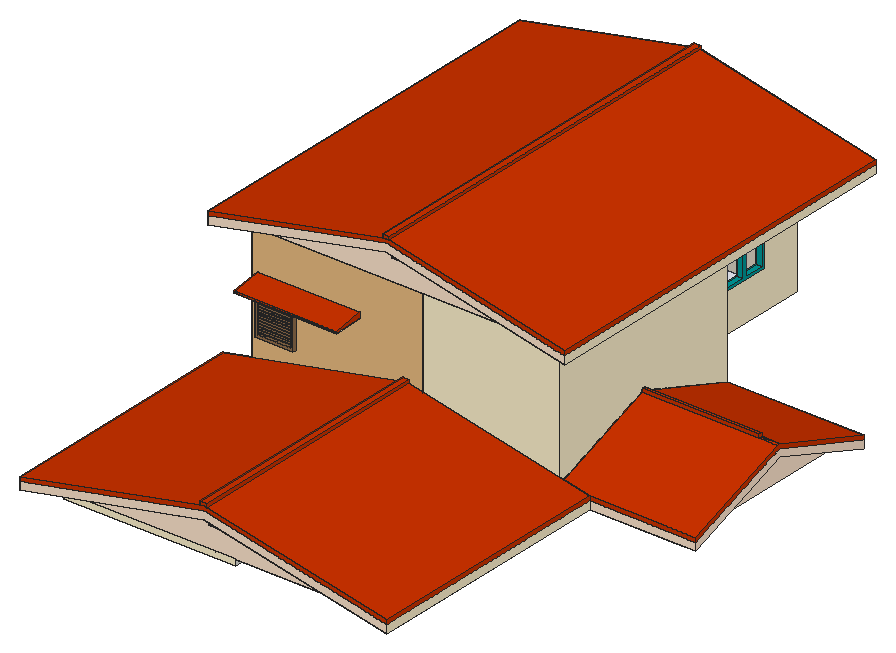
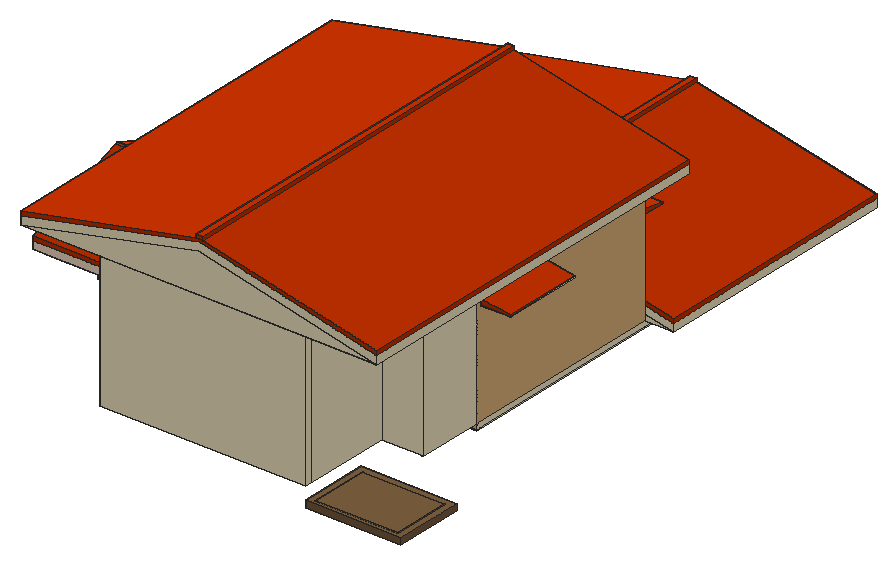
# SketchUp Ruby script. Lengths in inches.
U = 1.inch
M = Sketchup.active_model
def pt(a) = Geom::Point3d.new(a.map { |v| v * U })
def face(e, loops, mat)
  f = e.add_face(loops[0].map { |a| pt(a) })
  loops[1..].each { |l| e.add_face(l.map { |a| pt(a) }).erase! }
  f.material = f.back_material = mat if mat
  f
end
# faces: each face lists its corners as indices into pts; further lists are holes
def faces(e, pts, list, mat = nil) = list.each { |f| face(e, (f[0].is_a?(Array) ? f : [f]).map { |l| l.map { |i| pts[i] } }, mat) }
# xy, xz, yz: faces in a plane at the given z, y or x. An outline is a flat list of corners, or four numbers for a rectangle; further outlines are holes
def ring(l) = l.size == 4 ? [[l[0], l[1]], [l[2], l[1]], [l[2], l[3]], [l[0], l[3]]] : l.each_slice(2).to_a
def flat(e, list, mat, &to3) = list.each { |f| face(e, (f[0].is_a?(Array) ? f : [f]).map { |l| ring(l).map { |u, v| to3.(u, v) } }, mat) }
def xy(e, z, list, mat = nil) = flat(e, list, mat) { |x, y| [x, y, z] }
def xz(e, y, list, mat = nil) = flat(e, list, mat) { |x, z| [x, y, z] }
def yz(e, x, list, mat = nil) = flat(e, list, mat) { |y, z| [x, y, z] }
def lines(e, pts, list) = list.each { |a, b| e.add_line(pt(pts[a]), pt(pts[b])) }
# prism: a flat outline (further loops are holes) pulled along v
def prism(e, loops, v, mat = nil)
  f = face(e, loops, mat); d = Geom::Vector3d.new(v.map { |x| x * U })
  f.pushpull(f.normal.samedirection?(d) ? d.length : -d.length)
end
def box(e, o, s, mat = nil) = prism(e, [[o, [o[0] + s[0], o[1], o[2]], [o[0] + s[0], o[1] + s[1], o[2]], [o[0], o[1] + s[1], o[2]]]], [0, 0, s[2]], mat)
def at(x, y, z, deg = 0) = Geom::Transformation.translation(pt([x, y, z])) * Geom::Transformation.rotation(ORIGIN, Z_AXIS, deg.degrees)
def axes(o, x, y, z) = Geom::Transformation.new([*x, 0, *y, 0, *z, 0, *pt(o).to_a, 1])
def part(name) = M.definitions.add(name)
# library, detail: a bought-in or finely detailed component or shape, given as its bounding box
def library(name, o, s) = part(name).tap { |d| box(d.entities, o, s) }
def detail(e, o, s) = box(e.add_group.entities, o, s)
def put(e, d, t, mat = nil) = e.add_instance(d, t).tap { |i| i.material = mat if mat }
def group(e, t, mat = nil) = e.add_group.tap { |g| g.transformation = t; g.material = mat if mat }.entities
root = M.entities
M.materials.add("B06_Amber_Rust").color = [204, 51, 0]
M.materials.add("Brick_Stack_Bond_2K2").color = [186, 186, 186]
M.materials.add("C01_Vanilla_Cream").color = [255, 230, 206]
M.materials.add("D01_Frost_White").color = [255, 242, 206]
M.materials.add("Glass_Sky Reflection_1").color = [126, 138, 183]
M.materials["Glass_Sky Reflection_1"].alpha = 0.25
M.materials.add("H01_Misty_Ice1").color = [204, 255, 255]
M.materials.add("H07_Deep_Teal").color = [0, 153, 153]
M.materials.add("M09_Shadow_Night").color = [0, 0, 0]
M.materials.add("Plywood_01_1K").color = [125, 96, 64]
M.materials.add("Wood_Floor_01_1K1").color = [146, 111, 76]
M.materials.add("Wood_Floor_12_1K").color = [92, 75, 65]
M.materials.add("Wood_Veneer_15_1K").color = [103, 69, 45]
c1 = library("Group\#121",[0,30.0625,0],[1.875,126.125,1.875])
c2 = part("Group\#120")
box(c2.entities,[0,0,0],[9,239.6875,1],"Plywood_01_1K")
c3 = library("Group\#288",[0,0,0],[162,198.1,132])
c4 = part("Group\#269")
box(c4.entities,[0,0,0],[18.5,4.875,0.375],"H01_Misty_Ice1")
c5 = library("Group\#278",[0,-6,0],[72,6,96.9])
c6 = part("Group\#271")
xy(c6.entities,0,[[0,-3,42.6875,0]],"Wood_Floor_01_1K1")
xy(c6.entities,3,[[3,-3,39.6875,0]],"Wood_Floor_01_1K1")
xy(c6.entities,51.75,[[3,-3,39.6875,0]],"Wood_Floor_01_1K1")
xy(c6.entities,54.75,[[0,-3,42.6875,0]],"Wood_Floor_01_1K1")
xz(c6.entities,-3,[[[0,0,42.6875,54.75],[3,3,39.6875,51.75]],[3,3,39.6875,5.49],[3,6.39,39.6875,8.25],[3,9.15,39.6875,11.02],[3,11.92,39.6875,13.79],
  [3,14.6875,39.6875,16.55],[3,17.45,39.6875,19.32],[3,20.22,39.6875,22.09],[3,22.99,39.6875,24.85],[3,25.75,39.6875,27.62],
  [3,28.52,39.6875,30.39],[3,31.29,39.6875,33.15],[3,34.05,39.6875,35.92],[3,36.82,39.6875,38.6875],[3,39.59,39.6875,41.45],
  [3,42.35,39.6875,44.22],[3,45.12,39.6875,46.99],[3,47.89,39.6875,51.75]],"Wood_Floor_01_1K1")
xz(c6.entities,-3,[[3,5.49,39.6875,6.39],[3,8.25,39.6875,9.15],[3,11.02,39.6875,11.92],[3,13.79,39.6875,14.6875],[3,16.55,39.6875,17.45],
  [3,19.32,39.6875,20.22],[3,22.09,39.6875,22.99],[3,24.85,39.6875,25.75],[3,27.62,39.6875,28.52],[3,30.39,39.6875,31.29],
  [3,33.15,39.6875,34.05],[3,35.92,39.6875,36.82],[3,38.6875,39.6875,39.59],[3,41.45,39.6875,42.35],[3,44.22,39.6875,45.12],
  [3,46.99,39.6875,47.89]],"Wood_Veneer_15_1K")
xz(c6.entities,0,[[[0,0,42.6875,54.75],[3,3,39.6875,51.75]]],"Wood_Floor_01_1K1")
yz(c6.entities,0,[[-3,0,0,54.75]],"Wood_Floor_01_1K1")
yz(c6.entities,3,[[-3,3,0,51.75]],"Wood_Floor_01_1K1")
yz(c6.entities,39.6875,[[-3,3,0,51.75]],"Wood_Floor_01_1K1")
yz(c6.entities,42.6875,[[-3,0,0,54.75]],"Wood_Floor_01_1K1")
c7 = part("Group\#294")
xy(c7.entities,0,[[-83.875,-1.08,-21.5,12]],"B06_Amber_Rust")
xz(c7.entities,-1.08,[[-83.875,0.35,-21.5,1.68]],"B06_Amber_Rust")
xz(c7.entities,-1.08,[[-83.875,0,-21.5,0.35]],"D01_Frost_White")
xz(c7.entities,12,[[-83.875,0,-21.5,6]],"B06_Amber_Rust")
yz(c7.entities,-83.875,[[-1.08,0.35,-1.08,1.68,12,6,12,0.35]],"B06_Amber_Rust")
yz(c7.entities,-83.875,[[-1.08,0,12,0.35]],"D01_Frost_White")
yz(c7.entities,-21.5,[[-1.08,0.35,12,0.35,12,6,-1.08,1.68]],"B06_Amber_Rust")
yz(c7.entities,-21.5,[[-1.08,0,12,0.35]],"D01_Frost_White")
p = [[-83.875,-1.08,1.68],[-21.5,-1.08,1.68],[-21.5,12,6],[-83.875,12,6]]
faces(c7.entities,p,[[0,1,2,3]],"B06_Amber_Rust")
xy(root,138,[[1648.75,377.6875,1653.375,630.5625],[1653.375,377.6875,1810.75,386.6875],[1653.375,626.375,1653.375,630.5625,1648.75,630.5625,1648.75,635.6875,1810.75,635.6875,1810.75,626.375]],"D01_Frost_White")
xy(root,139,[[1926.75,626.6875,1939.75,635.6875]],"Brick_Stack_Bond_2K2")
xy(root,139,[[1648.75,377.6875,1653.375,630.5625],[1653.375,377.6875,1810.75,386.6875],[1653.375,626.375,1810.75,626.375,1810.75,635.6875,1648.75,635.6875,1648.75,630.5625,1653.375,630.5625]],"D01_Frost_White")
xy(root,139,[[[1584.5,740.6875,1674.5,806.6875],[1590.5,746.6875,1668.5,802.6875]],[1590.5,746.6875,1668.5,802.6875]],"Plywood_01_1K")
xy(root,139,[[1876.75,529.96,1882.75,533.5],[1876.75,533.5,1876.75,626.6875,1810.75,626.6875,1810.75,635.6875,1926.75,635.6875,1926.75,626.6875,1882.75,626.6875,1882.75,533.5]],"Wood_Floor_12_1K")
xy(root,144,[[1876.75,529.96,1882.75,626.6875]],"H01_Misty_Ice1")
xy(root,144,[[1810.75,626.6875,1876.75,635.6875],[1876.75,626.6875,1939.75,635.6875]],"Wood_Floor_12_1K")
xy(root,145,[[[1584.5,740.6875,1674.5,806.6875],[1590.5,746.6875,1668.5,802.6875]],[1590.5,746.6875,1668.5,802.6875]],"Plywood_01_1K")
xy(root,265,[[1876.75,529.96,1882.75,626.6875]],"H01_Misty_Ice1")
xz(root,377.6875,[[1648.75,138,1810.75,139]],"D01_Frost_White")
xz(root,386.6875,[[1653.375,138,1810.75,139]],"D01_Frost_White")
xz(root,529.96,[[1876.75,144,1882.75,265]],"H01_Misty_Ice1")
xz(root,529.96,[[1876.75,139,1882.75,142.54],[1876.75,142.54,1882.75,144]],"Wood_Floor_12_1K")
xz(root,626.375,[[1653.375,138,1810.75,139]],"D01_Frost_White")
xz(root,626.6875,[[1876.75,144,1882.75,265]],"H01_Misty_Ice1")
xz(root,626.6875,[[1810.75,139,1876.75,144],[1882.75,139,1939.75,144]],"Wood_Floor_12_1K")
xz(root,630.5625,[[1648.75,138,1653.375,139]],"D01_Frost_White")
xz(root,635.6875,[[1648.75,138,1810.75,139]],"D01_Frost_White")
xz(root,635.6875,[[1810.75,139,1939.75,144]],"Wood_Floor_12_1K")
xz(root,740.6875,[[1584.5,139,1674.5,145]],"Plywood_01_1K")
xz(root,802.6875,[[1590.5,139,1668.5,145]],"Plywood_01_1K")
xz(root,806.6875,[[1584.5,139,1674.5,145]],"Plywood_01_1K")
yz(root,1584.5,[[740.6875,139,806.6875,145]],"Plywood_01_1K")
yz(root,1590.5,[[746.6875,139,802.6875,145]],"Plywood_01_1K")
yz(root,1648.75,[[377.6875,138,630.5625,139],[630.5625,138,635.6875,139]],"D01_Frost_White")
yz(root,1653.375,[[386.6875,138,626.375,139],[626.375,138,630.5625,139]],"D01_Frost_White")
yz(root,1668.5,[[746.6875,139,802.6875,145]],"Plywood_01_1K")
yz(root,1674.5,[[740.6875,139,806.6875,145]],"Plywood_01_1K")
yz(root,1810.75,[[626.375,138,635.6875,139]],"D01_Frost_White")
yz(root,1810.75,[[377.6875,138,386.6875,139]],"Plywood_01_1K")
yz(root,1810.75,[[626.6875,139,635.6875,144]],"Wood_Floor_12_1K")
yz(root,1876.75,[[529.96,144,626.6875,265]],"H01_Misty_Ice1")
yz(root,1876.75,[[529.96,139,529.96,142.54,533.5,139],[533.5,139,529.96,142.54,529.96,144,626.6875,144,626.6875,139]],"Wood_Floor_12_1K")
yz(root,1882.75,[[529.96,144,626.6875,265]],"H01_Misty_Ice1")
yz(root,1882.75,[[529.96,139,533.5,139,529.96,142.54],[533.5,139,626.6875,139,626.6875,144,529.96,144,529.96,142.54]],"Wood_Floor_12_1K")
yz(root,1939.75,[[626.6875,139,635.6875,144]],"Wood_Floor_12_1K")
p = [[1746.46,517.53,124.68],[1746.56,517.91,123.72],[1746.46,517.53,138],[1882.75,533.5,139],[1876.75,533.5,139],[1876.75,529.96,142.54],
  [1882.75,529.96,142.54],[1648.75,437.6875,139],[1648.75,437.6875,138]]
faces(root,p,[[0,1,2]],"M09_Shadow_Night")
faces(root,p,[[3,4,5,6]],"Wood_Floor_12_1K")
lines(root,p,[[7,8]])
g1 = group(root,at(1648.75,224.6875,138))
xy(g1,-4.6875,[[9,0,153,144]],"Plywood_01_1K")
xy(g1,0,[[9,0,153,144]])
xz(g1,0,[[9,-4.6875,153,0]],"Plywood_01_1K")
xz(g1,144,[[9,-4.6875,153,0]])
yz(g1,9,[[0,-4.6875,144,0]],"Plywood_01_1K")
yz(g1,153,[[0,-4.6875,144,0]])
put(root,c1,at(1658.125,404.3125,135.875),"D01_Frost_White")
g2 = group(root,at(1648.75,215.6875,138))
xy(g2,0,[[0,0,162,162]])
xy(g2,6,[[0,0,162,162]],"D01_Frost_White")
xz(g2,0,[[0,0,162,6]],"D01_Frost_White")
xz(g2,162,[[0,0,162,6]])
yz(g2,0,[[0,0,162,6]],"D01_Frost_White")
yz(g2,162,[[0,0,162,6]])
g3 = group(root,at(1648.75,377.6875,139),"D01_Frost_White")
xy(g3,0,[[0,0,162,258]],"Plywood_01_1K")
xy(g3,5,[[0,0,162,258]])
xz(g3,0,[[0,0,162,5]])
xz(g3,258,[[0,0,162,5]])
yz(g3,0,[[0,0,258,5]])
yz(g3,162,[[0,0,258,5]])
put(g3,c2,axes([162,9,0],[-1,0,0],[0,1,0],[0,0,-1]))
put(g3,c2,axes([152.4,9,0],[-1,0,0],[0,1,0],[0,0,-1]))
put(g3,c2,axes([142.8,9,0],[-1,0,0],[0,1,0],[0,0,-1]))
put(g3,c2,axes([133.2,9,0],[-1,0,0],[0,1,0],[0,0,-1]))
put(g3,c2,axes([123.6,9,0],[-1,0,0],[0,1,0],[0,0,-1]))
put(g3,c2,axes([114,9,0],[-1,0,0],[0,1,0],[0,0,-1]))
put(g3,c2,axes([104.4,9,0],[-1,0,0],[0,1,0],[0,0,-1]))
put(g3,c2,axes([94.8,9,0],[-1,0,0],[0,1,0],[0,0,-1]))
put(g3,c2,axes([85.2,9,0],[-1,0,0],[0,1,0],[0,0,-1]))
put(g3,c2,axes([75.6,9,0],[-1,0,0],[0,1,0],[0,0,-1]))
put(g3,c2,axes([66,9,0],[-1,0,0],[0,1,0],[0,0,-1]))
put(g3,c2,axes([56.4,9,0],[-1,0,0],[0,1,0],[0,0,-1]))
put(g3,c2,axes([46.8,9,0],[-1,0,0],[0,1,0],[0,0,-1]))
put(g3,c2,axes([37.2,9,0],[-1,0,0],[0,1,0],[0,0,-1]))
put(g3,c2,axes([27.6,9,0],[-1,0,0],[0,1,0],[0,0,-1]))
put(g3,c2,axes([18,9,0],[-1,0,0],[0,1,0],[0,0,-1]))
put(root,c3,at(1648.75,437.6875,139),"D01_Frost_White")
g4 = group(root,at(2047.875,445.23,144),"C01_Vanilla_Cream")
xy(g4,0,[[-108.125,-7.54,3,190.46]])
xy(g4,50.08,[[-108.125,89.5,3,92.96]],"B06_Amber_Rust")
xz(g4,-7.54,[[-108.125,0,21,7.39]])
xz(g4,-7.54,[[-108.125,7.39,21,11.42]],"B06_Amber_Rust")
xz(g4,89.5,[[-108.125,46.71,3,50.08]],"B06_Amber_Rust")
xz(g4,92.96,[[-108.125,46.87,3,50.08]],"B06_Amber_Rust")
xz(g4,190.46,[[-108.125,0,21,7.39]])
xz(g4,190.46,[[-108.125,7.39,21,11.42]],"B06_Amber_Rust")
yz(g4,-108.125,[[-7.54,0,-7.54,7.39,91.46,44.26,190.46,7.39,190.46,0,91.46,36.87],[-7.54,0,91.46,36.87,190.46,0]])
yz(g4,-108.125,[[-7.54,7.39,-7.54,11.42,89.5,46.71,91.46,47.42,92.96,46.87,190.46,11.42,190.46,7.39,91.46,44.26],[89.5,46.71,89.5,50.08,92.96,50.08,92.96,46.87,91.46,47.42]],"B06_Amber_Rust")
yz(g4,3,[[89.5,46.71,91.46,47.42,92.96,46.87,92.96,50.08,89.5,50.08]],"B06_Amber_Rust")
yz(g4,3,[[-7.54,0,190.46,0,91.46,36]],"C01_Vanilla_Cream")
yz(g4,21,[[-7.54,7.39,91.46,43.39,190.46,7.39,190.46,11.42,92.96,46.87,91.46,47.42,89.5,46.71,-7.54,11.42]],"B06_Amber_Rust")
yz(g4,21,[[-7.54,0,91.46,36,190.46,0,190.46,7.39,91.46,43.39,-7.54,7.39]],"C01_Vanilla_Cream")
p = [[3,-7.54,0],[3,91.46,36],[21,91.46,36],[21,-7.54,0],[3,190.46,0],[21,190.46,0],
  [-108.125,-7.54,11.42],[21,-7.54,11.42],[21,89.5,46.71],[3,89.5,46.71],[-108.125,89.5,46.71],[-108.125,190.46,11.42],
  [-108.125,92.96,46.87],[3,92.96,46.87],[21,92.96,46.87],[21,190.46,11.42],[3,91.46,47.42],[-108.125,91.46,47.42],
  [21,91.46,47.42]]
faces(g4,p,[[0,1,2,3],[1,4,5,2]],"C01_Vanilla_Cream")
faces(g4,p,[[6,7,8,9,10],[11,12,13,14,15],[16,9,8,18],[13,16,18,14]],"B06_Amber_Rust")
faces(g4,p,[[9,16,17,10],[16,13,12,17]])
put(g4,c4,axes([3,86.53,20.34],[0,0.62857,0],[0,0,1],[0.66744,0,0]))
g5 = group(root,at(1876.75,437.6875,144),"D01_Frost_White")
xy(g5,0,[[-66,0,-66,6,54,6,54,189,0,189,0,198,63,198,63,0]])
xy(g5,100.25,[[-66,189,0,198]],"D01_Frost_White")
xy(g5,127,[[-66,0,63,0,63,198,-66,198,-66,189,54,189,54,6,-66,6]],"D01_Frost_White")
xz(g5,0,[[-66,0,63,127]])
xz(g5,6,[[-66,0,54,127]],"H01_Misty_Ice1")
xz(g5,189,[[0,0,54,0,54,127,-66,127,-66,100.25,0,100.25]],"H01_Misty_Ice1")
xz(g5,198,[[0,0,0,100.25,-66,100.25,-66,127,63,127,63,0]],"D01_Frost_White")
yz(g5,-66,[[0,0,6,127]])
yz(g5,-66,[[189,100.25,198,127]],"D01_Frost_White")
yz(g5,0,[[189,0,198,100.25]],"D01_Frost_White")
yz(g5,54,[[6,0,189,127]],"H01_Misty_Ice1")
yz(g5,63,[[0,0,198,127]],"D01_Frost_White")
g6 = group(root,at(1712.6875,635.6875,144),"D01_Frost_White")
xy(g6,0,[[-63.9375,0,0,63]])
xy(g6,0.1,[[-17.3125,57,54.14,63],[-24.3125,63,-17.3125,147]])
xy(g6,0.1,[[-58.5625,0,163.84,57]],"Plywood_01_1K")
xy(g6,36,[[163.84,67.8125,170.0625,115.8125]])
xy(g6,84,[[163.84,67.8125,170.0625,115.8125]])
xy(g6,97,[[-17.3125,57,54.14,63]])
xy(g6,127,[[-24.3125,63,-17.3125,147],[163.84,63,170.0625,147],[-24.3125,147,170.0625,153]])
xy(g6,129.375,[[-63.9375,0,-58.5625,0,-58.5625,57,163.84,57,163.84,0,170.0625,0,170.0625,63,-63.9375,63]])
xz(g6,0,[[-63.9375,0,6.22,0,6.22,0.1,-58.5625,0.1,-58.5625,129.375,-63.9375,129.375],[163.84,0,170.0625,129.375]])
xz(g6,0,[[6.22,0,163.84,0.1]],"Plywood_01_1K")
xz(g6,57,[[-58.5625,0.1,-17.3125,0.1,-17.3125,97,54.14,97,54.14,0.1,163.84,0.1,163.84,129.375,-58.5625,129.375]])
xz(g6,63,[[6.22,0,14.0625,0.1],[86.0625,0,163.84,0.1],[-63.9375,0.1,-24.3125,129.375],[-24.3125,127,-17.3125,129.375],[163.84,127,170.0625,129.375]])
xz(g6,63,[[-63.9375,0,0,0.1],[54.14,0.1,54.14,97,-17.3125,97,-17.3125,129.375,163.84,129.375,163.84,0.1]],"D01_Frost_White")
xz(g6,67.8125,[[163.84,36,170.0625,84]])
xz(g6,115.8125,[[163.84,36,170.0625,84]])
xz(g6,147,[[-24.3125,0.1,-17.3125,127],[-17.3125,0.1,0,127],[0,0.1,6.22,127],[6.22,0.1,163.84,127]])
xz(g6,153,[[0,0,0,0.1,-24.3125,0.1,-24.3125,127,170.0625,127,170.0625,0]])
yz(g6,-63.9375,[[0,0,63,129.375]],"D01_Frost_White")
yz(g6,-58.5625,[[0,0.1,57,129.375]])
yz(g6,-24.3125,[[63,0.1,147,127],[147,0.1,153,127]])
yz(g6,-17.3125,[[57,0.1,63,97],[63,0.1,147,127]])
yz(g6,54.14,[[57,0.1,63,97]])
yz(g6,163.84,[[0,0.1,57,129.375],[[63,0.1,147,127],[67.8125,36,115.8125,84]]])
yz(g6,170.0625,[[[63,0,153,127],[67.8125,36,115.8125,84]]])
yz(g6,170.0625,[[0,0,63,129.375]],"D01_Frost_White")
g7 = group(g6,at(164.0625,67.8125,36))
xy(g7,0,[[0,0,6,48]],"H07_Deep_Teal")
xy(g7,3,[[0,3,6,22.5],[0,25.5,6,45]],"H07_Deep_Teal")
xy(g7,45,[[0,3,6,22.5],[0,25.5,6,45]],"H07_Deep_Teal")
xy(g7,48,[[0,0,6,48]],"H07_Deep_Teal")
xz(g7,0,[[0,0,6,48]],"H07_Deep_Teal")
xz(g7,3,[[0,3,6,45]],"H07_Deep_Teal")
xz(g7,22.5,[[0,3,6,45]],"H07_Deep_Teal")
xz(g7,25.5,[[0,3,6,45]],"H07_Deep_Teal")
xz(g7,45,[[0,3,6,45]],"H07_Deep_Teal")
xz(g7,48,[[0,0,6,48]],"H07_Deep_Teal")
yz(g7,0,[[3,3,22.5,45],[25.5,3,45,45]],"Glass_Sky Reflection_1")
yz(g7,0,[[[0,0,48,48],[3,3,22.5,45],[25.5,3,45,45]]],"H07_Deep_Teal")
yz(g7,6,[[[0,0,48,48],[3,3,22.5,45],[25.5,3,45,45]]],"H07_Deep_Teal")
g8 = group(root,at(1634.96,215.83,144),"D01_Frost_White")
xy(g8,0,[[-13.2,0,333.29,221.86]])
xy(g8,50.08,[[156.63,-18,162.68,221.86]],"B06_Amber_Rust")
xz(g8,-18,[[-13.2,7.39,-5.28,9.04,160.05,43.39,325.37,9.04,333.29,7.39,333.29,11.42,162.68,46.87,160.05,47.42,156.63,46.71,-13.2,11.42],[156.63,46.71,160.05,47.42,162.68,46.87,162.68,50.08,156.63,50.08]],"B06_Amber_Rust")
xz(g8,-18,[[-13.2,0,160.05,36,333.29,0,333.29,7.39,325.37,9.04,160.05,43.39,-5.28,9.04,-13.2,7.39]],"C01_Vanilla_Cream")
xz(g8,0,[[-13.2,0,333.29,0,160.05,36]],"C01_Vanilla_Cream")
xz(g8,221.86,[[-13.2,0,-13.2,7.39,160.05,44.26,333.29,7.39,333.29,0,160.05,36.87],[-13.2,0,160.05,36.87,333.29,0]])
xz(g8,221.86,[[-13.2,7.39,-13.2,11.42,156.63,46.71,160.05,47.42,162.68,46.87,333.29,11.42,333.29,7.39,160.05,44.26],[156.63,46.71,156.63,50.08,162.68,50.08,162.68,46.87,160.05,47.42]],"B06_Amber_Rust")
yz(g8,-13.2,[[-18,0,221.86,7.39]])
yz(g8,-13.2,[[-18,7.39,221.86,11.42]],"B06_Amber_Rust")
yz(g8,156.63,[[-18,46.71,221.86,50.08]],"B06_Amber_Rust")
yz(g8,162.68,[[-18,46.87,221.86,50.08]],"B06_Amber_Rust")
yz(g8,333.29,[[-18,0,221.86,7.39]])
yz(g8,333.29,[[-18,7.39,221.86,11.42]],"B06_Amber_Rust")
p = [[-13.2,0,0],[160.05,0,36],[160.05,-18,36],[-13.2,-18,0],[333.29,0,0],[333.29,-18,0],
  [-13.2,221.86,11.42],[-13.2,-18,11.42],[156.63,-18,46.71],[156.63,221.86,46.71],[333.29,221.86,11.42],[162.68,221.86,46.87],
  [162.68,-18,46.87],[333.29,-18,11.42],[160.05,-18,47.42],[160.05,221.86,47.42]]
faces(g8,p,[[0,1,2,3],[1,4,5,2]],"C01_Vanilla_Cream")
faces(g8,p,[[6,7,8,9],[10,11,12,13]],"B06_Amber_Rust")
faces(g8,p,[[8,14,15,9],[14,12,11,15]])
put(g8,c4,axes([151.42,0,20.34],[1.09998,0,0],[0,0,1],[0,-1.36952,0]))
put(root,c5,at(1694.82,698.6875,144))
put(root,c6,axes([1654.21,437.6875,181],[0.84,0,0],[0,1,0],[0,0,0.87671]))
put(root,c7,axes([1908.31,778.49,228],[0,1,0],[-2.13,0,0],[0,0,1]),"D01_Frost_White")
g9 = group(root,at(1772.75,412.13,229),"D01_Frost_White")
xy(g9,0,[[-118.55,-2.3,-21.5,25.56]],"B06_Amber_Rust")
xz(g9,-2.3,[[-118.55,0.35,-21.5,1.68]],"B06_Amber_Rust")
xz(g9,-2.3,[[-118.55,0,-21.5,0.35]],"D01_Frost_White")
xz(g9,25.56,[[-118.55,0,-21.5,6]],"B06_Amber_Rust")
yz(g9,-118.55,[[-2.3,0.35,-2.3,1.68,25.56,6,25.56,0.35]],"B06_Amber_Rust")
yz(g9,-118.55,[[-2.3,0,25.56,0.35]],"D01_Frost_White")
yz(g9,-21.5,[[-2.3,0.35,25.56,0.35,25.56,6,-2.3,1.68]],"B06_Amber_Rust")
yz(g9,-21.5,[[-2.3,0,25.56,0.35]],"D01_Frost_White")
p = [[-118.55,-2.3,1.68],[-21.5,-2.3,1.68],[-21.5,25.56,6],[-118.55,25.56,6]]
faces(g9,p,[[0,1,2,3]],"B06_Amber_Rust")
g10 = group(root,at(1623.19,535.1875,241.99))
xy(g10,0,[[-2.3,19.9375,25.56,96.0625]],"B06_Amber_Rust")
xz(g10,19.9375,[[-2.3,0.35,25.56,0.35,25.56,6,-2.3,1.68]],"B06_Amber_Rust")
xz(g10,19.9375,[[-2.3,0,25.56,0.35]],"D01_Frost_White")
xz(g10,96.0625,[[-2.3,0.35,-2.3,1.68,25.56,6,25.56,0.35]],"B06_Amber_Rust")
xz(g10,96.0625,[[-2.3,0,25.56,0.35]],"D01_Frost_White")
yz(g10,-2.3,[[19.9375,0.35,96.0625,1.68]],"B06_Amber_Rust")
yz(g10,-2.3,[[19.9375,0,96.0625,0.35]],"D01_Frost_White")
yz(g10,25.56,[[19.9375,0,96.0625,6]],"B06_Amber_Rust")
p = [[-2.3,96.0625,1.68],[-2.3,19.9375,1.68],[25.56,19.9375,6],[25.56,96.0625,6]]
faces(g10,p,[[0,1,2,3]],"B06_Amber_Rust")
g11 = group(root,at(1633.75,438.125,271),"D01_Frost_White")
xy(g11,0,[[-12.86,0,324.62,350.5625]])
xy(g11,50.08,[[152.55,-18,158.44,350.5625]],"B06_Amber_Rust")
xz(g11,-18,[[-12.86,7.39,-5.14,9.04,155.88,43.39,316.9,9.04,324.62,7.39,324.62,11.42,158.44,46.87,155.88,47.42,152.55,46.71,-12.86,11.42],[152.55,46.71,155.88,47.42,158.44,46.87,158.44,50.08,152.55,50.08]],"B06_Amber_Rust")
xz(g11,-18,[[-12.86,0,155.88,36,324.62,0,324.62,7.39,316.9,9.04,155.88,43.39,-5.14,9.04,-12.86,7.39]],"C01_Vanilla_Cream")
xz(g11,0,[[-12.86,0,324.62,0,155.88,36]],"C01_Vanilla_Cream")
xz(g11,350.5625,[[-12.86,0,-12.86,7.39,155.88,44.26,324.62,7.39,324.62,0,155.88,36.87],[-12.86,0,155.88,36.87,324.62,0]])
xz(g11,350.5625,[[-12.86,7.39,-12.86,11.42,152.55,46.71,155.88,47.42,158.44,46.87,324.62,11.42,324.62,7.39,155.88,44.26],[152.55,46.71,152.55,50.08,158.44,50.08,158.44,46.87,155.88,47.42]],"B06_Amber_Rust")
yz(g11,-12.86,[[-18,0,350.5625,7.39]])
yz(g11,-12.86,[[-18,7.39,350.5625,11.42]],"B06_Amber_Rust")
yz(g11,152.55,[[-18,46.71,350.5625,50.08]],"B06_Amber_Rust")
yz(g11,158.44,[[-18,46.87,350.5625,50.08]],"B06_Amber_Rust")
yz(g11,324.62,[[-18,0,350.5625,7.39]])
yz(g11,324.62,[[-18,7.39,350.5625,11.42]],"B06_Amber_Rust")
p = [[-12.86,0,0],[155.88,0,36],[155.88,-18,36],[-12.86,-18,0],[324.62,0,0],[324.62,-18,0],
  [-12.86,350.5625,11.42],[-12.86,-18,11.42],[152.55,-18,46.71],[152.55,350.5625,46.71],[324.62,350.5625,11.42],[158.44,350.5625,46.87],
  [158.44,-18,46.87],[324.62,-18,11.42],[155.88,-18,47.42],[155.88,350.5625,47.42]]
faces(g11,p,[[0,1,2,3],[1,4,5,2]],"C01_Vanilla_Cream")
faces(g11,p,[[6,7,8,9],[10,11,12,13]],"B06_Amber_Rust")
faces(g11,p,[[8,14,15,9],[14,12,11,15]])
put(g11,c4,axes([147.48,0,20.34],[1.07136,0,0],[0,0,1],[0,-2.16397,0]))
